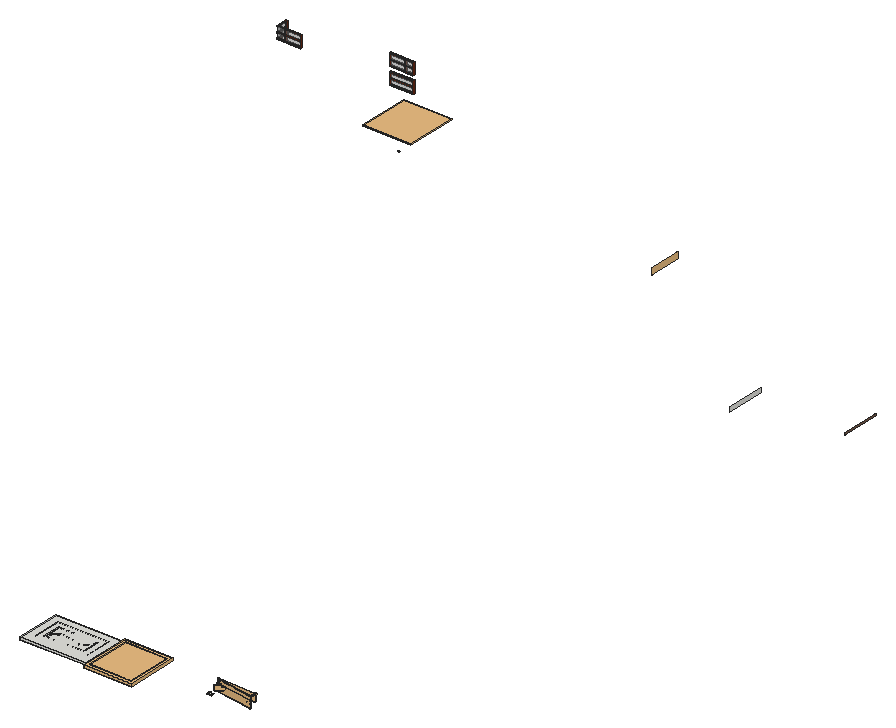
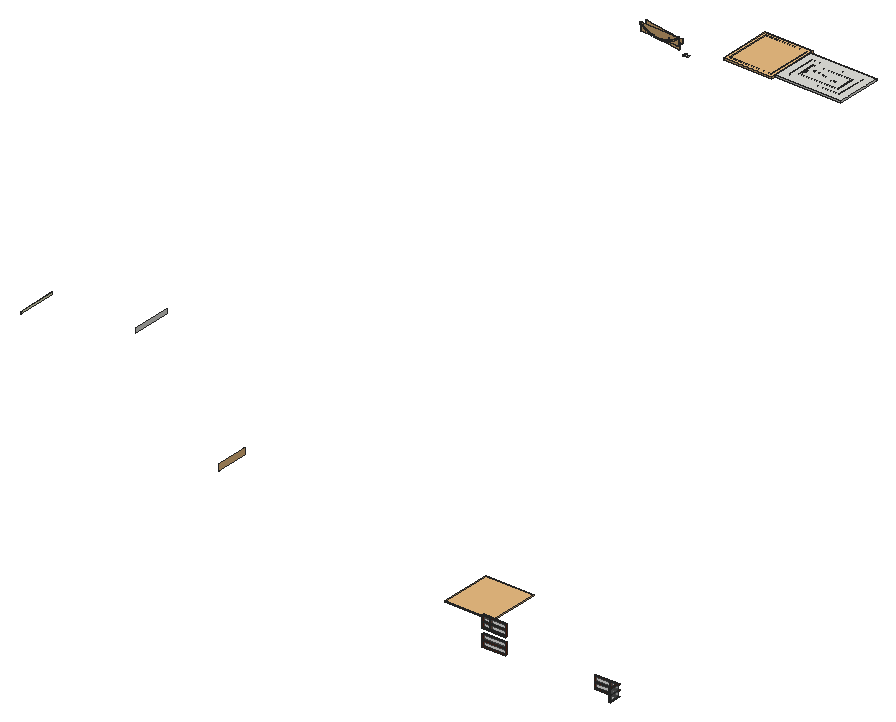
# SketchUp Ruby script. Lengths in inches.
U = 1.inch
M = Sketchup.active_model
def pt(a) = Geom::Point3d.new(a.map { |v| v * U })
def face(e, loops, mat)
  f = e.add_face(loops[0].map { |a| pt(a) })
  loops[1..].each { |l| e.add_face(l.map { |a| pt(a) }).erase! }
  f.material = f.back_material = mat if mat
  f
end
# faces: each face lists its corners as indices into pts; further lists are holes
def faces(e, pts, list, mat = nil) = list.each { |f| face(e, (f[0].is_a?(Array) ? f : [f]).map { |l| l.map { |i| pts[i] } }, mat) }
# xy, xz, yz: faces in a plane at the given z, y or x. An outline is a flat list of corners, or four numbers for a rectangle; further outlines are holes
def ring(l) = l.size == 4 ? [[l[0], l[1]], [l[2], l[1]], [l[2], l[3]], [l[0], l[3]]] : l.each_slice(2).to_a
def flat(e, list, mat, &to3) = list.each { |f| face(e, (f[0].is_a?(Array) ? f : [f]).map { |l| ring(l).map { |u, v| to3.(u, v) } }, mat) }
def xy(e, z, list, mat = nil) = flat(e, list, mat) { |x, y| [x, y, z] }
def xz(e, y, list, mat = nil) = flat(e, list, mat) { |x, z| [x, y, z] }
def yz(e, x, list, mat = nil) = flat(e, list, mat) { |y, z| [x, y, z] }
def lines(e, pts, list) = list.each { |a, b| e.add_line(pt(pts[a]), pt(pts[b])) }
# prism: a flat outline (further loops are holes) pulled along v
def prism(e, loops, v, mat = nil)
  f = face(e, loops, mat); d = Geom::Vector3d.new(v.map { |x| x * U })
  f.pushpull(f.normal.samedirection?(d) ? d.length : -d.length)
end
def box(e, o, s, mat = nil) = prism(e, [[o, [o[0] + s[0], o[1], o[2]], [o[0] + s[0], o[1] + s[1], o[2]], [o[0], o[1] + s[1], o[2]]]], [0, 0, s[2]], mat)
def at(x, y, z, deg = 0) = Geom::Transformation.translation(pt([x, y, z])) * Geom::Transformation.rotation(ORIGIN, Z_AXIS, deg.degrees)
def axes(o, x, y, z) = Geom::Transformation.new([*x, 0, *y, 0, *z, 0, *pt(o).to_a, 1])
def part(name) = M.definitions.add(name)
# library, detail: a bought-in or finely detailed component or shape, given as its bounding box
def library(name, o, s) = part(name).tap { |d| box(d.entities, o, s) }
def detail(e, o, s) = box(e.add_group.entities, o, s)
def put(e, d, t, mat = nil) = e.add_instance(d, t).tap { |i| i.material = mat if mat }
def group(e, t, mat = nil) = e.add_group.tap { |g| g.transformation = t; g.material = mat if mat }.entities
root = M.entities
M.materials.add("02 - Default1").color = [198, 154, 113]
M.materials.add("1").color = [234, 234, 196]
M.materials.add("3").color = [118, 89, 74]
M.materials.add("Emissive").color = [114, 114, 114]
M.materials.add("Window Frame").color = [102, 40, 20]
M.materials.add("[Color_004]").color = [142, 142, 142]
M.materials.add("[Color_007]").color = [58, 58, 58]
M.materials.add("[Color_B17]").color = [102, 40, 20]
M.materials.add("[Color_C12]").color = [153, 91, 30]
M.materials.add("[Translucent_Glass_Gray]").color = [128, 128, 128]
M.materials["[Translucent_Glass_Gray]"].alpha = 0.5
c1 = library("Group\#99",[0,0,0],[124,134,3.84])
c2 = library("Group\#86",[0,0,0],[154,144,7.49])
c3 = library("Group\#67",[-88.79,0.67,-41.3125],[0.99,6.14,4.87])
c4 = library("Group\#64",[-88.79,21.34,-41.3125],[0.99,6.53,4.87])
c5 = library("Lichterkette",[-8.5625,-0.06,-0.42],[198.07,2.65,35.24])
c6 = library("New Assembly\#10",[-473.6,471.11,165.93],[120.62,2.52,31.03])
c7 = part("Component\#432")
box(c7.entities,[-13.78,0,0],[13.78,19.88,0.79])
c8 = library("Componente",[-1.36,-1.19,-8.45],[2.52,2.52,8.45])
c9 = library("Grupo22\#1",[-472.57,-0.06,139.2],[0.26,472.56,57.77])
c10 = part("New Assembly\#9")
put(c10.entities,c8,at(-472.44,0,196.85,90))
put(c10.entities,c8,at(-472.44,23.62,185.95,90))
put(c10.entities,c8,at(-472.44,472.44,196.85,90))
put(c10.entities,c8,at(-472.44,448.82,185.95,90))
put(c10.entities,c8,at(-472.44,47.24,175.78,90))
put(c10.entities,c8,at(-472.44,70.87,167.1,90))
put(c10.entities,c8,at(-472.44,94.49,159.8,90))
put(c10.entities,c8,at(-472.44,118.11,153.19,90))
put(c10.entities,c8,at(-472.44,141.73,148.55,90))
put(c10.entities,c8,at(-472.44,165.35,144.53,90))
put(c10.entities,c8,at(-472.44,188.98,141.78,90))
put(c10.entities,c8,at(-472.44,212.6,140.25,90))
put(c10.entities,c8,at(-472.44,236.22,139.34,90))
put(c10.entities,c8,at(-472.44,259.84,140.25,90))
put(c10.entities,c8,at(-472.44,283.46,141.78,90))
put(c10.entities,c8,at(-472.44,307.09,144.53,90))
put(c10.entities,c8,at(-472.44,330.71,148.55,90))
put(c10.entities,c8,at(-472.44,354.33,153.19,90))
put(c10.entities,c8,at(-472.44,377.95,159.8,90))
put(c10.entities,c8,at(-472.44,401.57,167.1,90))
put(c10.entities,c8,at(-472.44,425.2,175.78,90))
put(c10.entities,c9,at(0,0,0))
c11 = part("Group\#331")
xy(c11.entities,0,[[0,0,0.82,6.2]],"1")
xy(c11.entities,114.11,[[0,0,0.82,6.2]],"1")
xz(c11.entities,0,[[0,0,0.82,114.11]],"1")
xz(c11.entities,6.2,[[0,0,0.82,114.11]],"1")
yz(c11.entities,0,[[0,0,6.2,114.11]],"1")
yz(c11.entities,0.82,[[0,0,6.2,114.11]],"3")
c12 = part("Group\#330")
put(c12.entities,c11,axes([-0.82,0,0],[1,0,0],[0,1.45243,0],[0,0,1]),"1")
c13 = library("Group\#222",[0,0,0],[5,19.46,126.79])
c14 = library("Group\#84",[0,0,0],[154,144,1.49])
c15 = part("Group\#37")
xz(c15.entities,0,[[0,0,67.32,15.06]],"[Translucent_Glass_Gray]")
c16 = part("Group\#23")
xy(c16.entities,0,[[0,0,67.32,15.94]],"[Translucent_Glass_Gray]")
c17 = part("Group\#35")
xz(c17.entities,0,[[0,0,44.29,15.94]],"[Translucent_Glass_Gray]")
put(root,c1,at(1543.51,380.85,122.95))
put(root,c2,at(1533.51,524.85,119.3,-90))
g1 = group(root,at(1337.47,514.85,126.79))
xy(g1,-6,[[[0,-134,196.04,0],[24.75,-109.25,171.29,-24.75]]])
xy(g1,-3.42,[[22.8,-111.2,171.29,-109.25],[171.29,-111.2,173.24,-22.8],[22.8,-109.25,24.75,-22.8],[[39.67,-94.33,39.67,-39.67,156.37,-39.67,155.99,-45.96,154.48,-52.08,151.875,-57.82,148.28,-63,143.8,-67.4375,138.59,-70.99,132.82,-73.53,126.6875,-74.99,120.39,-75.31,114.14,-74.48,108.15,-72.53,102.6,-69.53,96.83,-66.32,90.62,-64.07,84.125,-62.85,77.52,-62.67,70.97,-63.56,64.65,-65.48,58.72,-68.39,53.33,-72.21,48.62,-76.84,44.71,-82.16,41.7,-88.05],[42.17,-81.63,42.57,-80.84,46.72,-75.2,51.72,-70.28,57.4375,-66.23,63.73,-63.15,70.4375,-61.11,77.38,-60.17,84.39,-60.35,91.28,-61.65,97.87,-64.03,103.81,-67.34,109.14,-70.22,114.7,-72.03,120.49,-72.8,126.33,-72.5,132.02,-71.15,137.37,-68.79,142.2,-65.5,146.35,-61.38,149.69,-56.58,152.1,-51.26,153.51,-45.58,153.71,-42.17,42.17,-42.17]],[[39.67,-94.33,41.7,-88.05,44.71,-82.16,48.62,-76.84,53.33,-72.21,58.72,-68.39,64.65,-65.48,70.97,-63.56,77.52,-62.67,84.125,-62.85,90.62,-64.07,96.83,-66.32,102.6,-69.53,108.15,-72.53,114.14,-74.48,120.39,-75.31,126.6875,-74.99,132.82,-73.53,138.59,-70.99,143.8,-67.4375,148.28,-63,151.875,-57.82,154.48,-52.08,155.99,-45.96,156.37,-39.67,156.37,-94.33],[41.7,-92.85,154.89,-92.85,154.89,-54.76,153.17,-58.56,149.41,-63.96,144.74,-68.58,139.31,-72.29,133.29,-74.94,126.9,-76.46,120.33,-76.8,113.8125,-75.93,107.56,-73.9,101.89,-70.83,96.21,-67.67,90.23,-65.5,83.97,-64.32,77.6,-64.16,71.29,-65.01,65.2,-66.86,59.48,-69.67,54.28,-73.35,49.74,-77.8125,45.97,-82.94,43.07,-88.61]],
  [24.75,-24.75,171.29,-22.8]])
xy(g1,-1.22,[[42.17,-81.63,42.17,-42.17,153.71,-42.17,153.51,-45.58,152.1,-51.26,149.69,-56.58,146.35,-61.38,142.2,-65.5,137.37,-68.79,132.02,-71.15,126.33,-72.5,120.49,-72.8,114.7,-72.03,109.14,-70.22,103.81,-67.34,97.87,-64.03,91.28,-61.65,84.39,-60.35,77.38,-60.17,70.4375,-61.11,63.73,-63.15,57.4375,-66.23,51.72,-70.28,46.72,-75.2,42.57,-80.84]])
xy(g1,-0.85,[[[22.8,-111.2,173.24,-22.8],[39.67,-94.33,156.37,-39.67]]])
xy(g1,0,[[0,-134,196.04,0]])
xz(g1,-134,[[0,-6,196.04,0]])
xz(g1,-111.2,[[22.8,-3.42,173.24,-0.85]],"Emissive")
xz(g1,-109.25,[[24.75,-6,171.29,-3.42]])
xz(g1,-94.33,[[39.67,-3.42,156.37,-0.85]])
xz(g1,-92.85,[[41.7,-3.42,154.89,-1.4]])
xz(g1,-42.17,[[42.17,-3.42,153.71,-1.22]])
xz(g1,-39.67,[[39.67,-3.42,156.37,-0.85]])
xz(g1,-24.75,[[24.75,-6,171.29,-3.42]])
xz(g1,-22.8,[[22.8,-3.42,173.24,-0.85]],"Emissive")
xz(g1,0,[[0,-6,196.04,0]])
yz(g1,0,[[-134,-6,0,0]])
yz(g1,22.8,[[-111.2,-3.42,-22.8,-0.85]],"Emissive")
yz(g1,24.75,[[-109.25,-6,-24.75,-3.42]])
yz(g1,39.67,[[-94.33,-3.42,-39.67,-0.85]])
yz(g1,42.17,[[-81.63,-3.42,-42.17,-1.22]])
yz(g1,154.89,[[-92.85,-3.42,-54.76,-1.4]])
yz(g1,156.37,[[-94.33,-3.42,-39.67,-0.85]])
yz(g1,171.29,[[-109.25,-6,-24.75,-3.42]])
yz(g1,173.24,[[-111.2,-3.42,-22.8,-0.85]],"Emissive")
yz(g1,196.04,[[-134,-6,0,0]])
p = [[41.7,-92.85,-3.42],[43.07,-88.61,-3.42],[43.07,-88.61,-1.4],[41.7,-92.85,-1.4],[45.97,-82.94,-3.42],[45.97,-82.94,-1.4],
  [49.74,-77.8125,-3.42],[49.74,-77.8125,-1.4],[42.57,-80.84,-3.42],[42.17,-81.63,-3.42],[42.17,-81.63,-1.22],[42.57,-80.84,-1.22],
  [46.72,-75.2,-3.42],[46.72,-75.2,-1.22],[54.28,-73.35,-3.42],[54.28,-73.35,-1.4],[113.8125,-75.93,-3.42],[120.33,-76.8,-3.42],
  [120.33,-76.8,-1.4],[113.8125,-75.93,-1.4],[126.9,-76.46,-3.42],[126.9,-76.46,-1.4],[133.29,-74.94,-3.42],[133.29,-74.94,-1.4],
  [107.56,-73.9,-3.42],[107.56,-73.9,-1.4],[51.72,-70.28,-3.42],[51.72,-70.28,-1.22],[139.31,-72.29,-3.42],[139.31,-72.29,-1.4],
  [101.89,-70.83,-3.42],[101.89,-70.83,-1.4],[59.48,-69.67,-3.42],[59.48,-69.67,-1.4],[120.49,-72.8,-3.42],[114.7,-72.03,-3.42],
  [114.7,-72.03,-1.22],[120.49,-72.8,-1.22],[126.33,-72.5,-3.42],[126.33,-72.5,-1.22],[132.02,-71.15,-3.42],[132.02,-71.15,-1.22],
  [144.74,-68.58,-3.42],[144.74,-68.58,-1.4],[109.14,-70.22,-3.42],[109.14,-70.22,-1.22],[137.37,-68.79,-3.42],[137.37,-68.79,-1.22],
  [96.21,-67.67,-3.42],[96.21,-67.67,-1.4],[57.4375,-66.23,-3.42],[57.4375,-66.23,-1.22],[103.81,-67.34,-3.42],[103.81,-67.34,-1.22],
  [65.2,-66.86,-3.42],[65.2,-66.86,-1.4],[142.2,-65.5,-3.42],[142.2,-65.5,-1.22],[149.41,-63.96,-3.42],[149.41,-63.96,-1.4],
  [90.23,-65.5,-3.42],[90.23,-65.5,-1.4],[97.87,-64.03,-3.42],[97.87,-64.03,-1.22],[71.29,-65.01,-3.42],[71.29,-65.01,-1.4],
  [63.73,-63.15,-3.42],[63.73,-63.15,-1.22],[83.97,-64.32,-3.42],[83.97,-64.32,-1.4],[146.35,-61.38,-3.42],[146.35,-61.38,-1.22],
  [77.6,-64.16,-3.42],[77.6,-64.16,-1.4],[91.28,-61.65,-3.42],[91.28,-61.65,-1.22],[153.17,-58.56,-3.42],[153.17,-58.56,-1.4],
  [70.4375,-61.11,-3.42],[70.4375,-61.11,-1.22],[84.39,-60.35,-3.42],[84.39,-60.35,-1.22],[149.69,-56.58,-3.42],[149.69,-56.58,-1.22],
  [77.38,-60.17,-3.42],[77.38,-60.17,-1.22],[154.89,-54.76,-3.42],[154.89,-54.76,-1.4],[152.1,-51.26,-3.42],[152.1,-51.26,-1.22],
  [153.51,-45.58,-3.42],[153.51,-45.58,-1.22],[153.71,-42.17,-3.42],[153.71,-42.17,-1.22]]
faces(g1,p,[[0,1,2,3],[1,4,5,2],[4,6,7,5],[8,9,10,11],[12,8,11,13],[6,14,15,7],[16,17,18,19],[17,20,21,18],
  [20,22,23,21],[24,16,19,25],[26,12,13,27],[22,28,29,23],[30,24,25,31],[14,32,33,15],[34,35,36,37],[38,34,37,39],
  [40,38,39,41],[28,42,43,29],[35,44,45,36],[46,40,41,47],[48,30,31,49],[50,26,27,51],[44,52,53,45],[32,54,55,33],
  [56,46,47,57],[42,58,59,43],[60,48,49,61],[52,62,63,53],[54,64,65,55],[66,50,51,67],[68,60,61,69],[70,56,57,71],
  [64,72,73,65],[72,68,69,73],[62,74,75,63],[58,76,77,59],[78,66,67,79],[74,80,81,75],[82,70,71,83],[84,78,79,85],
  [80,84,85,81],[76,86,87,77],[88,82,83,89],[90,88,89,91],[92,90,91,93]],"Emissive")
g2 = group(root,at(1533.51,448.8,108.52))
detail(g2,[-7.8125,-1.23,-4.27],[0.08,0.64,0.5])
g3 = group(root,at(1533.51,448.8,108.52))
prism(g3,[[[-7.73,0.02,-3.89],[-7.73,0.02,-3.77],[-7.73,-0.54,-3.77],[-7.73,-0.54,-3.89],[-7.73,-0.36,-3.89],[-7.73,-0.36,-4.27],[-7.73,-0.17,-4.27],[-7.73,-0.17,-3.89]]],[-0.09,0,0],"[Color_004]")
g4 = group(root,at(1533.51,448.8,108.52))
prism(g4,[[[-7.73,18.74,-8.96],[-7.73,18.74,-2.44],[-7.7,18.74,-2.06],[-7.625,18.74,-1.6875],[-7.5,18.74,-1.33],[-7.33,18.74,-1.01],[-7.12,18.74,-0.72],[-6.87,18.74,-0.47],[-6.59,18.74,-0.27],[-6.29,18.74,-0.12],[-5.97,18.74,-0.03],[-5.65,18.74,0],[-5.65,18.74,-0.12],[-5.96,18.74,-0.15],[-6.26,18.74,-0.24],[-6.54,18.74,-0.375],[-6.81,18.74,-0.57],[-7.04,18.74,-0.8],[-7.24,18.74,-1.08],[-7.41,18.74,-1.39],[-7.53,18.74,-1.72],[-7.6,18.74,-2.08],[-7.62,18.74,-2.44],[-7.62,18.74,-8.96]]],[0,-37.47,0])
g5 = group(root,at(1533.51,448.8,108.52))
xy(g5,-12.74,[[-1.73,-18.76,0,18.76]])
xy(g5,-2.26,[[-0.93,-15.67,-0.73,-11.93],[-0.64,-15.67,-0.43,-11.93],[-0.35,-15.67,-0.14,-11.93],[-0.93,-11.73,-0.73,-7.99],[-0.64,-11.73,-0.43,-7.99],
  [-0.35,-11.73,-0.14,-7.99],[-0.93,-7.79,-0.73,-4.04],[-0.64,-7.79,-0.43,-4.04],[-0.35,-7.79,-0.14,-4.04],[-0.93,-3.84,-0.73,-0.1],
  [-0.64,-3.84,-0.43,-0.1],[-0.35,-3.84,-0.14,-0.1],[-0.93,0.1,-0.73,3.84],[-0.64,0.1,-0.43,3.84],[-0.35,0.1,-0.14,3.84],
  [-0.93,4.04,-0.73,7.79],[-0.64,4.04,-0.43,7.79],[-0.35,4.04,-0.14,7.79],[-0.93,7.99,-0.73,11.73],[-0.64,7.99,-0.43,11.73],
  [-0.35,7.99,-0.14,11.73],[-0.93,11.93,-0.73,15.67],[-0.64,11.93,-0.43,15.67],[-0.35,11.93,-0.14,15.67]])
xy(g5,0,[[[-1.73,-18.76,0,18.76],[-0.93,4.04,-0.93,11.73,-0.73,11.73,-0.73,7.99,-0.93,7.99,-0.93,7.79,-0.73,7.79,-0.73,4.04],[-0.35,4.04,-0.35,7.79,-0.14,7.79,-0.14,7.99,-0.35,7.99,-0.35,11.73,-0.14,11.73,-0.14,4.04],[-0.64,11.93,-0.43,15.67],[-0.35,11.93,-0.14,15.67],[-0.93,11.93,-0.73,15.67],[-0.93,-15.67,-0.73,-11.93],[-0.35,-15.67,-0.14,-11.93],[-0.64,-15.67,-0.43,-11.93],[-0.64,4.04,-0.43,7.79],[-0.35,-7.79,-0.14,-4.04],[-0.64,-7.79,-0.43,-4.04],[-0.93,-7.79,-0.73,-4.04],[-0.64,7.99,-0.43,11.73],[-0.64,0.1,-0.43,3.84],[-0.35,0.1,-0.14,3.84],[-0.93,0.1,-0.73,3.84],[-0.35,-11.73,-0.14,-7.99],[-0.93,-11.73,-0.73,-7.99],[-0.93,-3.84,-0.73,-0.1],[-0.64,-3.84,-0.43,-0.1],[-0.35,-3.84,-0.14,-0.1],[-0.64,-11.73,-0.43,-7.99]]])
xz(g5,-18.76,[[-1.73,-12.74,0,0]])
xz(g5,-15.67,[[-0.93,-2.26,-0.73,0],[-0.64,-2.26,-0.43,0],[-0.35,-2.26,-0.14,0]])
xz(g5,-11.93,[[-0.93,-2.26,-0.73,0],[-0.64,-2.26,-0.43,0],[-0.35,-2.26,-0.14,0]])
xz(g5,-11.73,[[-0.93,-2.26,-0.73,0],[-0.64,-2.26,-0.43,0],[-0.35,-2.26,-0.14,0]])
xz(g5,-7.99,[[-0.93,-2.26,-0.73,0],[-0.64,-2.26,-0.43,0],[-0.35,-2.26,-0.14,0]])
xz(g5,-7.79,[[-0.93,-2.26,-0.73,0],[-0.64,-2.26,-0.43,0],[-0.35,-2.26,-0.14,0]])
xz(g5,-4.04,[[-0.93,-2.26,-0.73,0],[-0.64,-2.26,-0.43,0],[-0.35,-2.26,-0.14,0]])
xz(g5,-3.84,[[-0.93,-2.26,-0.73,0],[-0.64,-2.26,-0.43,0],[-0.35,-2.26,-0.14,0]])
xz(g5,-0.1,[[-0.93,-2.26,-0.73,0],[-0.64,-2.26,-0.43,0],[-0.35,-2.26,-0.14,0]])
xz(g5,0.1,[[-0.93,-2.26,-0.73,0],[-0.64,-2.26,-0.43,0],[-0.35,-2.26,-0.14,0]])
xz(g5,3.84,[[-0.93,-2.26,-0.73,0],[-0.64,-2.26,-0.43,0],[-0.35,-2.26,-0.14,0]])
xz(g5,4.04,[[-0.93,-2.26,-0.73,0],[-0.64,-2.26,-0.43,0],[-0.35,-2.26,-0.14,0]])
xz(g5,7.79,[[-0.93,-2.26,-0.73,0],[-0.64,-2.26,-0.43,0],[-0.35,-2.26,-0.14,0]])
xz(g5,7.99,[[-0.93,-2.26,-0.73,0],[-0.64,-2.26,-0.43,0],[-0.35,-2.26,-0.14,0]])
xz(g5,11.73,[[-0.93,-2.26,-0.73,0],[-0.64,-2.26,-0.43,0],[-0.35,-2.26,-0.14,0]])
xz(g5,11.93,[[-0.93,-2.26,-0.73,0],[-0.64,-2.26,-0.43,0],[-0.35,-2.26,-0.14,0]])
xz(g5,15.67,[[-0.93,-2.26,-0.73,0],[-0.64,-2.26,-0.43,0],[-0.35,-2.26,-0.14,0]])
xz(g5,18.76,[[-1.73,-12.74,0,0]])
yz(g5,-1.73,[[-18.76,-12.74,18.76,0]])
yz(g5,-0.93,[[-15.67,-2.26,-11.93,0],[-11.73,-2.26,-7.99,0],[-7.79,-2.26,-4.04,0],[-3.84,-2.26,-0.1,0],[0.1,-2.26,3.84,0],
  [4.04,-2.26,7.79,0],[7.99,-2.26,11.73,0],[11.93,-2.26,15.67,0]])
yz(g5,-0.73,[[-15.67,-2.26,-11.93,0],[-11.73,-2.26,-7.99,0],[-7.79,-2.26,-4.04,0],[-3.84,-2.26,-0.1,0],[0.1,-2.26,3.84,0],
  [4.04,-2.26,7.79,0],[7.99,-2.26,11.73,0],[11.93,-2.26,15.67,0]])
yz(g5,-0.64,[[-15.67,-2.26,-11.93,0],[-11.73,-2.26,-7.99,0],[-7.79,-2.26,-4.04,0],[-3.84,-2.26,-0.1,0],[0.1,-2.26,3.84,0],
  [4.04,-2.26,7.79,0],[7.99,-2.26,11.73,0],[11.93,-2.26,15.67,0]])
yz(g5,-0.43,[[-15.67,-2.26,-11.93,0],[-11.73,-2.26,-7.99,0],[-7.79,-2.26,-4.04,0],[-3.84,-2.26,-0.1,0],[0.1,-2.26,3.84,0],
  [4.04,-2.26,7.79,0],[7.99,-2.26,11.73,0],[11.93,-2.26,15.67,0]])
yz(g5,-0.35,[[-15.67,-2.26,-11.93,0],[-11.73,-2.26,-7.99,0],[-7.79,-2.26,-4.04,0],[-3.84,-2.26,-0.1,0],[0.1,-2.26,3.84,0],
  [4.04,-2.26,7.79,0],[7.99,-2.26,11.73,0],[11.93,-2.26,15.67,0]])
yz(g5,-0.14,[[-15.67,-2.26,-11.93,0],[-11.73,-2.26,-7.99,0],[-7.79,-2.26,-4.04,0],[-3.84,-2.26,-0.1,0],[0.1,-2.26,3.84,0],
  [4.04,-2.26,7.79,0],[7.99,-2.26,11.73,0],[11.93,-2.26,15.67,0]])
yz(g5,0,[[-18.76,-12.74,18.76,0]])
g6 = group(root,at(1533.51,448.8,108.52))
xy(g6,-12.74,[[-5.65,-18.76,-1.73,-15.875],[-5.65,15.875,-1.73,18.76]])
xy(g6,-9.91,[[-7.03,-15.875,-1.73,15.875]])
xy(g6,-9.7,[[-7.03,-3.48,-6.93,3.48]])
xy(g6,-9.07,[[-7.03,-3.48,-6.93,3.48]])
xy(g6,-8.96,[[-7.73,-18.76,-7.62,-15.875],[-7.62,-15.875,-7.03,15.875],[-7.73,15.875,-7.62,18.76]])
xy(g6,0,[[-5.65,-18.76,-1.73,18.76]])
xz(g6,-18.76,[[-5.65,-12.74,-1.73,-12.74,-1.73,0,-5.65,0,-5.65,-0.12,-5.96,-0.15,-6.26,-0.24,-6.54,-0.375,-6.81,-0.57,-7.04,-0.8,-7.24,-1.08,-7.41,-1.39,-7.53,-1.72,-7.6,-2.08,-7.62,-2.44,-7.62,-8.96,-7.73,-8.96,-7.73,-10.29,-7.7,-10.68,-7.625,-11.05,-7.5,-11.4,-7.33,-11.73,-7.12,-12.02,-6.87,-12.27,-6.59,-12.47,-6.29,-12.62,-5.97,-12.71]])
xz(g6,-15.875,[[-5.65,-12.74,-5.97,-12.71,-6.29,-12.62,-6.59,-12.47,-6.87,-12.27,-7.12,-12.02,-7.33,-11.73,-7.5,-11.4,-7.625,-11.05,-7.7,-10.68,-7.73,-10.29,-7.73,-8.96,-7.03,-8.96,-7.03,-9.91,-1.73,-9.91,-1.73,-12.74]])
xz(g6,-3.48,[[-7.03,-9.7,-6.93,-9.07]])
xz(g6,3.48,[[-7.03,-9.7,-6.93,-9.07]])
xz(g6,15.875,[[-5.65,-12.74,-1.73,-12.74,-1.73,-9.91,-7.03,-9.91,-7.03,-8.96,-7.73,-8.96,-7.73,-10.29,-7.7,-10.68,-7.625,-11.05,-7.5,-11.4,-7.33,-11.73,-7.12,-12.02,-6.87,-12.27,-6.59,-12.47,-6.29,-12.62,-5.97,-12.71]])
xz(g6,18.76,[[-5.65,-12.74,-5.97,-12.71,-6.29,-12.62,-6.59,-12.47,-6.87,-12.27,-7.12,-12.02,-7.33,-11.73,-7.5,-11.4,-7.625,-11.05,-7.7,-10.68,-7.73,-10.29,-7.73,-8.96,-7.62,-8.96,-7.62,-2.44,-7.6,-2.08,-7.53,-1.72,-7.41,-1.39,-7.24,-1.08,-7.04,-0.8,-6.81,-0.57,-6.54,-0.375,-6.26,-0.24,-5.96,-0.15,-5.65,-0.12,-5.65,0,-1.73,0,-1.73,-12.74]])
yz(g6,-7.73,[[-18.76,-10.29,-15.875,-8.96],[15.875,-10.29,18.76,-8.96]])
yz(g6,-7.62,[[-18.76,-8.96,18.76,-2.44]])
yz(g6,-7.03,[[[-15.875,-9.91,15.875,-8.96],[-3.48,-9.7,3.48,-9.07]]])
yz(g6,-6.93,[[-3.48,-9.7,3.48,-9.07]],"[Color_007]")
yz(g6,-5.65,[[-18.76,-0.12,18.76,0]])
yz(g6,-1.73,[[-18.76,-12.74,-15.875,-12.74,-15.875,-9.91,15.875,-9.91,15.875,-12.74,18.76,-12.74,18.76,0,-18.76,0]])
p = [[-6.29,-18.76,-12.62],[-6.29,-15.875,-12.62],[-5.97,-15.875,-12.71],[-5.97,-18.76,-12.71],[-5.65,-15.875,-12.74],[-5.65,-18.76,-12.74],
  [-6.29,15.875,-12.62],[-6.29,18.76,-12.62],[-5.97,18.76,-12.71],[-5.97,15.875,-12.71],[-5.65,18.76,-12.74],[-5.65,15.875,-12.74],
  [-6.59,-15.875,-12.47],[-6.59,-18.76,-12.47],[-6.59,15.875,-12.47],[-6.59,18.76,-12.47],[-6.87,-18.76,-12.27],[-6.87,-15.875,-12.27],
  [-6.87,15.875,-12.27],[-6.87,18.76,-12.27],[-7.12,-18.76,-12.02],[-7.12,-15.875,-12.02],[-7.12,15.875,-12.02],[-7.12,18.76,-12.02],
  [-7.33,-18.76,-11.73],[-7.33,-15.875,-11.73],[-7.33,15.875,-11.73],[-7.33,18.76,-11.73],[-7.5,-18.76,-11.4],[-7.5,-15.875,-11.4],
  [-7.5,15.875,-11.4],[-7.5,18.76,-11.4],[-7.625,-15.875,-11.05],[-7.625,-18.76,-11.05],[-7.625,15.875,-11.05],[-7.625,18.76,-11.05],
  [-7.7,-18.76,-10.68],[-7.7,-15.875,-10.68],[-7.7,15.875,-10.68],[-7.7,18.76,-10.68],[-7.73,-18.76,-10.29],[-7.73,-15.875,-10.29],
  [-7.73,15.875,-10.29],[-7.73,18.76,-10.29],[-7.62,18.76,-2.44],[-7.62,-18.76,-2.44],[-7.6,-18.76,-2.08],[-7.6,18.76,-2.08],
  [-7.53,-18.76,-1.72],[-7.53,18.76,-1.72],[-7.41,18.76,-1.39],[-7.41,-18.76,-1.39],[-7.24,-18.76,-1.08],[-7.24,18.76,-1.08],
  [-7.04,-18.76,-0.8],[-7.04,18.76,-0.8],[-6.81,-18.76,-0.57],[-6.81,18.76,-0.57],[-6.54,-18.76,-0.375],[-6.54,18.76,-0.375],
  [-6.26,18.76,-0.24],[-6.26,-18.76,-0.24],[-5.96,-18.76,-0.15],[-5.96,18.76,-0.15],[-5.65,-18.76,-0.12],[-5.65,18.76,-0.12]]
faces(g6,p,[[0,1,2,3],[4,5,3,2],[6,7,8,9],[10,11,9,8],[12,1,0,13],[6,14,15,7],[12,13,16,17],[15,14,18,19],
  [20,21,17,16],[22,23,19,18],[21,20,24,25],[23,22,26,27],[28,29,25,24],[30,31,27,26],[32,29,28,33],[30,34,35,31],
  [32,33,36,37],[35,34,38,39],[40,41,37,36],[42,43,39,38],[44,45,46,47],[48,49,47,46],[50,49,48,51],[50,51,52,53],
  [54,55,53,52],[55,54,56,57],[58,59,57,56],[60,59,58,61],[60,61,62,63],[64,65,63,62]])
g7 = group(root,at(1533.51,448.8,108.52))
xy(g7,-12.375,[[-5.58,-15.875,-3.67,15.875]])
xy(g7,-10.42,[[-7.25,-15.875,-7,-9.1],[-7.25,-8.85,-7,4.71],[-7.25,4.95,-7,15.875]])
xy(g7,-9.91,[[-7,-15.875,-3.67,-15.875,-3.67,15.875,-7,15.875,-7,4.95,-7.25,4.95,-7.25,4.71,-7,4.71,-7,-8.85,-7.25,-8.85,-7.25,-9.1,-7,-9.1]])
xz(g7,-15.875,[[-5.58,-12.375,-3.67,-12.375,-3.67,-9.91,-7,-9.91,-7,-10.42,-7.25,-10.42,-7.24,-10.46,-7.23,-10.73,-7.17,-11.02,-7.07,-11.31,-6.93,-11.57,-6.76,-11.8,-6.5625,-12,-6.34,-12.16,-6.1,-12.28,-5.84,-12.35]])
xz(g7,-9.1,[[-7.25,-10.42,-7,-9.91]])
xz(g7,-8.85,[[-7.25,-10.42,-7,-9.91]])
xz(g7,4.71,[[-7.25,-10.42,-7,-9.91]])
xz(g7,4.95,[[-7.25,-10.42,-7,-9.91]])
xz(g7,15.875,[[-5.58,-12.375,-5.84,-12.35,-6.1,-12.28,-6.34,-12.16,-6.5625,-12,-6.76,-11.8,-6.93,-11.57,-7.07,-11.31,-7.17,-11.02,-7.23,-10.73,-7.24,-10.46,-7.25,-10.42,-7,-10.42,-7,-9.91,-3.67,-9.91,-3.67,-12.375]])
yz(g7,-7.25,[[-9.1,-10.42,-8.85,-9.91],[4.71,-10.42,4.95,-9.91]])
yz(g7,-7,[[-15.875,-10.42,-9.1,-9.91],[-8.85,-10.42,4.71,-9.91],[4.95,-10.42,15.875,-9.91]],"[Color_007]")
yz(g7,-3.67,[[-15.875,-12.375,15.875,-9.91]])
p = [[-5.58,15.875,-12.375],[-5.58,-15.875,-12.375],[-5.84,-15.875,-12.35],[-5.84,15.875,-12.35],[-6.34,15.875,-12.16],[-6.1,15.875,-12.28],
  [-6.1,-15.875,-12.28],[-6.34,-15.875,-12.16],[-6.5625,-15.875,-12],[-6.5625,15.875,-12],[-6.76,-15.875,-11.8],[-6.76,15.875,-11.8],
  [-6.93,-15.875,-11.57],[-6.93,15.875,-11.57],[-7.07,-15.875,-11.31],[-7.07,15.875,-11.31],[-7.17,15.875,-11.02],[-7.17,-15.875,-11.02],
  [-7.23,-15.875,-10.73],[-7.23,15.875,-10.73],[-7.24,-15.875,-10.46],[-7.24,-9.1,-10.46],[-7.24,-8.85,-10.46],[-7.24,4.71,-10.46],
  [-7.24,4.95,-10.46],[-7.24,15.875,-10.46],[-7.25,15.875,-10.42],[-7.25,-15.875,-10.42],[-7.25,-9.1,-10.42],[-7.25,-8.85,-10.42],
  [-7.25,4.71,-10.42],[-7.25,4.95,-10.42]]
faces(g7,p,[[0,1,2,3],[4,5,6,7],[6,5,3,2],[4,7,8,9],[10,11,9,8],[11,10,12,13],[14,15,13,12],[16,15,14,17],
  [16,17,18,19],[18,20,21,22,23,24,25,19]])
faces(g7,p,[[26,25,24,23,22,21,20,27,28,29,30,31]],"[Color_C12]")
put(root,c3,axes([1533.51,448.8,108.52],[0.088,0,0],[0,0.10336,0],[0,0,0.10336]))
g8 = group(root,at(1533.51,448.8,108.52))
prism(g8,[[[-7.726,1.3,-4.27],[-7.726,1.487,-4.27],[-7.726,1.213,-3.794],[-7.726,1.206,-3.785],[-7.726,1.197,-3.777],[-7.726,1.187,-3.772],[-7.726,1.176,-3.768],[-7.726,1.165,-3.767],[-7.726,1.04,-3.767],[-7.726,1.028,-3.768],[-7.726,1.017,-3.772],[-7.726,1.007,-3.777],[-7.726,0.999,-3.785],[-7.726,0.992,-3.794],[-7.726,0.718,-4.27],[-7.726,0.904,-4.27],[-7.726,0.965,-4.164],[-7.726,1.239,-4.164]],[[-7.726,1.191,-4.08],[-7.726,1.014,-4.08],[-7.726,1.102,-3.927]]],[-0.088,0,0],"[Color_004]")
g9 = group(root,at(1533.51,448.8,108.52))
detail(g9,[-7.8125,1.46,-4.27],[0.08,0.67,0.5])
put(root,c4,axes([1533.51,448.8,108.52],[0.088,0,0],[0,0.10336,0],[0,0,0.10336]))
put(root,c5,axes([1821.67,513.93,93.78],[0.57877,-0.0831,0],[-0.0091,-0.06335,0],[0,0,0.568]))
put(root,c5,axes([1822.75,514.27,106.12],[0.57267,-0.08482,0],[-0.00938,-0.06331,0],[0,0,0.568]))
put(root,c6,axes([2023.74,390.17,37.17],[0.25961,0.12734,0],[-0.17615,0.35913,0],[0,0,0.4]))
put(root,c7,axes([1793.64,504.67,82.12],[0,-0.69,0],[0.69,0,0],[0,0,0.69]))
put(root,c10,axes([1932.48,703.84,48],[0,0.4,0],[-0.24297,0,0],[0,0,0.4]))
g10 = group(root,at(1942.8125,2264.52,114.11))
yz(g10,0,[[0,0,114.54,12.68]])
put(root,c12,axes([2215.32,2470.24,108.07],[1,0,0],[0,0,0.67033],[0,-1.0271,0]),"02 - Default1")
put(root,c13,axes([1389.45,2763.18,107.33],[0.12,0,0],[0,0,1],[0,-0.75975,0]))
g11 = group(root,at(527.48,2794.13,79.75))
detail(g11,[1.46,7.73,-4.27],[0.67,0.08,0.5])
g12 = group(root,at(527.48,2794.13,79.75),"[Color_004]")
prism(g12,[[[-1.4375,7.73,-4.27],[-1.27,7.73,-4.27],[-1.4,7.73,-3.77],[-1.61,7.73,-3.77],[-1.73,7.73,-4.11],[-1.84,7.73,-3.77],[-2.04,7.73,-3.77],[-2.17,7.73,-4.27],[-2.01,7.73,-4.27],[-1.92,7.73,-3.93],[-1.82,7.73,-4.27],[-1.64,7.73,-4.27],[-1.53,7.73,-3.92]]],[0,0.09,0],"[Color_004]")
put(root,c4,axes([527.48,2794.13,79.75],[0,-0.088,0],[0.10336,0,0],[0,0,0.10336]))
put(root,c3,axes([527.48,2794.13,79.75],[0,-0.088,0],[0.10336,0,0],[0,0,0.10336]))
g13 = group(root,at(527.48,2794.13,79.75))
detail(g13,[-2.86,7.73,-4.27],[0.65,0.08,0.5])
g14 = group(root,at(527.48,2794.13,79.75))
prism(g14,[[[0.02,7.73,-3.89],[0.02,7.73,-3.77],[-0.54,7.73,-3.77],[-0.54,7.73,-3.89],[-0.36,7.73,-3.89],[-0.36,7.73,-4.27],[-0.17,7.73,-4.27],[-0.17,7.73,-3.89]]],[0,0.09,0],"[Color_004]")
g15 = group(root,at(527.48,2794.13,79.75))
prism(g15,[[[1.3,7.726,-4.27],[1.487,7.726,-4.27],[1.213,7.726,-3.794],[1.206,7.726,-3.785],[1.197,7.726,-3.777],[1.187,7.726,-3.772],[1.176,7.726,-3.768],[1.165,7.726,-3.767],[1.04,7.726,-3.767],[1.028,7.726,-3.768],[1.017,7.726,-3.772],[1.007,7.726,-3.777],[0.999,7.726,-3.785],[0.992,7.726,-3.794],[0.718,7.726,-4.27],[0.904,7.726,-4.27],[0.965,7.726,-4.164],[1.239,7.726,-4.164]],[[1.191,7.726,-4.08],[1.014,7.726,-4.08],[1.102,7.726,-3.927]]],[0,0.088,0],"[Color_004]")
g16 = group(root,at(527.48,2794.13,79.75))
detail(g16,[-1.23,7.73,-4.27],[0.64,0.08,0.5])
g17 = group(root,at(527.48,2794.13,79.75))
prism(g17,[[[-0.82,7.73,-4.08],[-0.77,7.73,-3.96],[-1.15,7.73,-3.96],[-1.23,7.73,-4.08]]],[0,0.09,0],"[Color_004]")
put(root,c14,axes([578.85,2937.05,120.79],[0,-1,0],[-1,0,0],[0,0,-1]))
g18 = group(root,at(334.5,3008.87,94))
put(g18,c15,at(1.77,1.57,1.77))
g19 = group(g18,at(0,4.33,-29.53))
prism(g19,[[[70.87,-4.33,29.53],[70.87,-4.33,64.96],[0,-4.33,64.96],[0,-4.33,29.53]],[[69.09,-4.33,46.36],[69.09,-4.33,31.3],[1.77,-4.33,31.3],[1.77,-4.33,46.36]],[[69.09,-4.33,63.1875],[69.09,-4.33,48.13],[1.77,-4.33,48.13],[1.77,-4.33,63.1875]]],[0,4.33,0],"[Color_B17]")
put(g18,c16,axes([1.77,1.57,17.72],[1,0,0],[0,0,1],[0,-1,0]))
g20 = group(root,at(334.5,3008.87,143.65))
put(g20,c15,at(1.77,1.57,1.77))
g21 = group(g20,at(0,4.33,-29.53))
xy(g21,29.53,[[0,-4.33,70.87,0]],"Window Frame")
xy(g21,31.3,[[1.77,-4.33,46.0625,0],[47.83,-4.33,69.09,0]],"Window Frame")
xy(g21,46.36,[[1.77,-4.33,46.0625,0],[47.83,-4.33,69.09,0]],"Window Frame")
xy(g21,48.13,[[1.77,-4.33,46.0625,0],[47.83,-4.33,69.09,0]],"Window Frame")
xy(g21,63.1875,[[1.77,-4.33,46.0625,0],[47.83,-4.33,69.09,0]],"Window Frame")
xy(g21,64.96,[[0,-4.33,70.87,0]],"Window Frame")
xz(g21,-4.33,[[[0,29.53,70.87,64.96],[1.77,31.3,46.0625,46.36],[1.77,48.13,46.0625,63.1875],[47.83,31.3,69.09,46.36],[47.83,48.13,69.09,63.1875]]],"Window Frame")
xz(g21,0,[[[0,29.53,70.87,64.96],[1.77,31.3,69.09,31.3,69.09,46.36,47.83,46.36,47.83,31.3,46.0625,31.3,46.0625,46.36,1.77,46.36],[1.77,48.13,46.0625,48.13,46.0625,63.1875,47.83,63.1875,47.83,48.13,69.09,48.13,69.09,63.1875,1.77,63.1875]]],"Window Frame")
yz(g21,0,[[-4.33,29.53,0,64.96]],"Window Frame")
yz(g21,1.77,[[-4.33,31.3,0,46.36],[-4.33,48.13,0,63.1875]],"Window Frame")
yz(g21,46.0625,[[-4.33,31.3,0,46.36],[-4.33,48.13,0,63.1875]],"Window Frame")
yz(g21,47.83,[[-4.33,31.3,0,46.36],[-4.33,48.13,0,63.1875]],"Window Frame")
yz(g21,69.09,[[-4.33,31.3,0,46.36],[-4.33,48.13,0,63.1875]],"Window Frame")
yz(g21,70.87,[[-4.33,29.53,0,64.96]],"Window Frame")
put(g20,c16,axes([1.77,1.57,17.72],[1,0,0],[0,0,1],[0,-1,0]))
g22 = group(root,at(0,3008.3,99.49))
put(g22,c17,at(25.49,1.57,17.72))
g23 = group(g22,at(1.57,1.57,-27.76))
xz(g23,0,[[0,29.53,22.15,44.59]],"[Translucent_Glass_Gray]")
yz(g23,0,[[0,29.53,29.92,44.59]],"[Translucent_Glass_Gray]")
g24 = group(g22,at(0,0,-29.53))
xy(g24,29.53,[[0,0,0,33.27,4.33,33.27,4.33,4.33,71.56,4.33,71.56,0]],"[Color_B17]")
xy(g24,31.3,[[0,0,23.72,0,23.72,4.33,4.33,4.33,4.33,31.5,0,31.5],[25.49,0,69.79,4.33]],"[Color_B17]")
xy(g24,46.36,[[0,0,0,31.5,4.33,31.5,4.33,4.33,23.72,4.33,23.72,0],[25.49,0,69.79,4.33]],"[Color_B17]")
xy(g24,48.13,[[0,0,23.72,0,23.72,4.33,4.33,4.33,4.33,31.5,0,31.5],[25.49,0,69.79,4.33]],"[Color_B17]")
xy(g24,63.1875,[[0,0,0,31.5,4.33,31.5,4.33,4.33,23.72,4.33,23.72,0],[25.49,0,69.79,4.33]],"[Color_B17]")
xy(g24,64.96,[[0,0,71.56,0,71.56,4.33,4.33,4.33,4.33,33.27,0,33.27]],"[Color_B17]")
xz(g24,0,[[[0,29.53,71.56,29.53,71.56,64.96,0,64.96,0,63.1875,23.72,63.1875,23.72,48.13,0,48.13,0,46.36,23.72,46.36,23.72,31.3,0,31.3],[25.49,31.3,69.79,46.36],[25.49,48.13,69.79,63.1875]]],"[Color_B17]")
xz(g24,4.33,[[[4.33,29.53,4.33,31.3,23.72,31.3,23.72,46.36,4.33,46.36,4.33,48.13,23.72,48.13,23.72,63.1875,4.33,63.1875,4.33,64.96,71.56,64.96,71.56,29.53],[25.49,31.3,69.79,46.36],[25.49,48.13,69.79,63.1875]]],"[Color_B17]")
xz(g24,31.5,[[0,31.3,4.33,46.36],[0,48.13,4.33,63.1875]],"[Color_B17]")
xz(g24,33.27,[[0,29.53,4.33,64.96]],"[Color_B17]")
yz(g24,0,[[0,29.53,0,31.3,31.5,31.3,31.5,46.36,0,46.36,0,48.13,31.5,48.13,31.5,63.1875,0,63.1875,0,64.96,33.27,64.96,33.27,29.53]],"[Color_B17]")
yz(g24,4.33,[[4.33,29.53,33.27,29.53,33.27,64.96,4.33,64.96,4.33,63.1875,31.5,63.1875,31.5,48.13,4.33,48.13,4.33,46.36,31.5,46.36,31.5,31.3,4.33,31.3]],"[Color_B17]")
yz(g24,23.72,[[0,31.3,4.33,46.36],[0,48.13,4.33,63.1875]],"[Color_B17]")
yz(g24,25.49,[[0,31.3,4.33,46.36],[0,48.13,4.33,63.1875]],"[Color_B17]")
yz(g24,69.79,[[0,31.3,4.33,46.36],[0,48.13,4.33,63.1875]],"[Color_B17]")
yz(g24,71.56,[[0,29.53,4.33,64.96]],"[Color_B17]")
g25 = group(g22,at(1.57,1.57,17.72))
xz(g25,0,[[0,0,22.15,15.94]],"[Translucent_Glass_Gray]")
yz(g25,0,[[0,0,29.92,15.94]],"[Translucent_Glass_Gray]")
g26 = group(g22,at(25.49,1.57,1.77))
xz(g26,0,[[0,0,44.29,15.06]],"[Translucent_Glass_Gray]")
